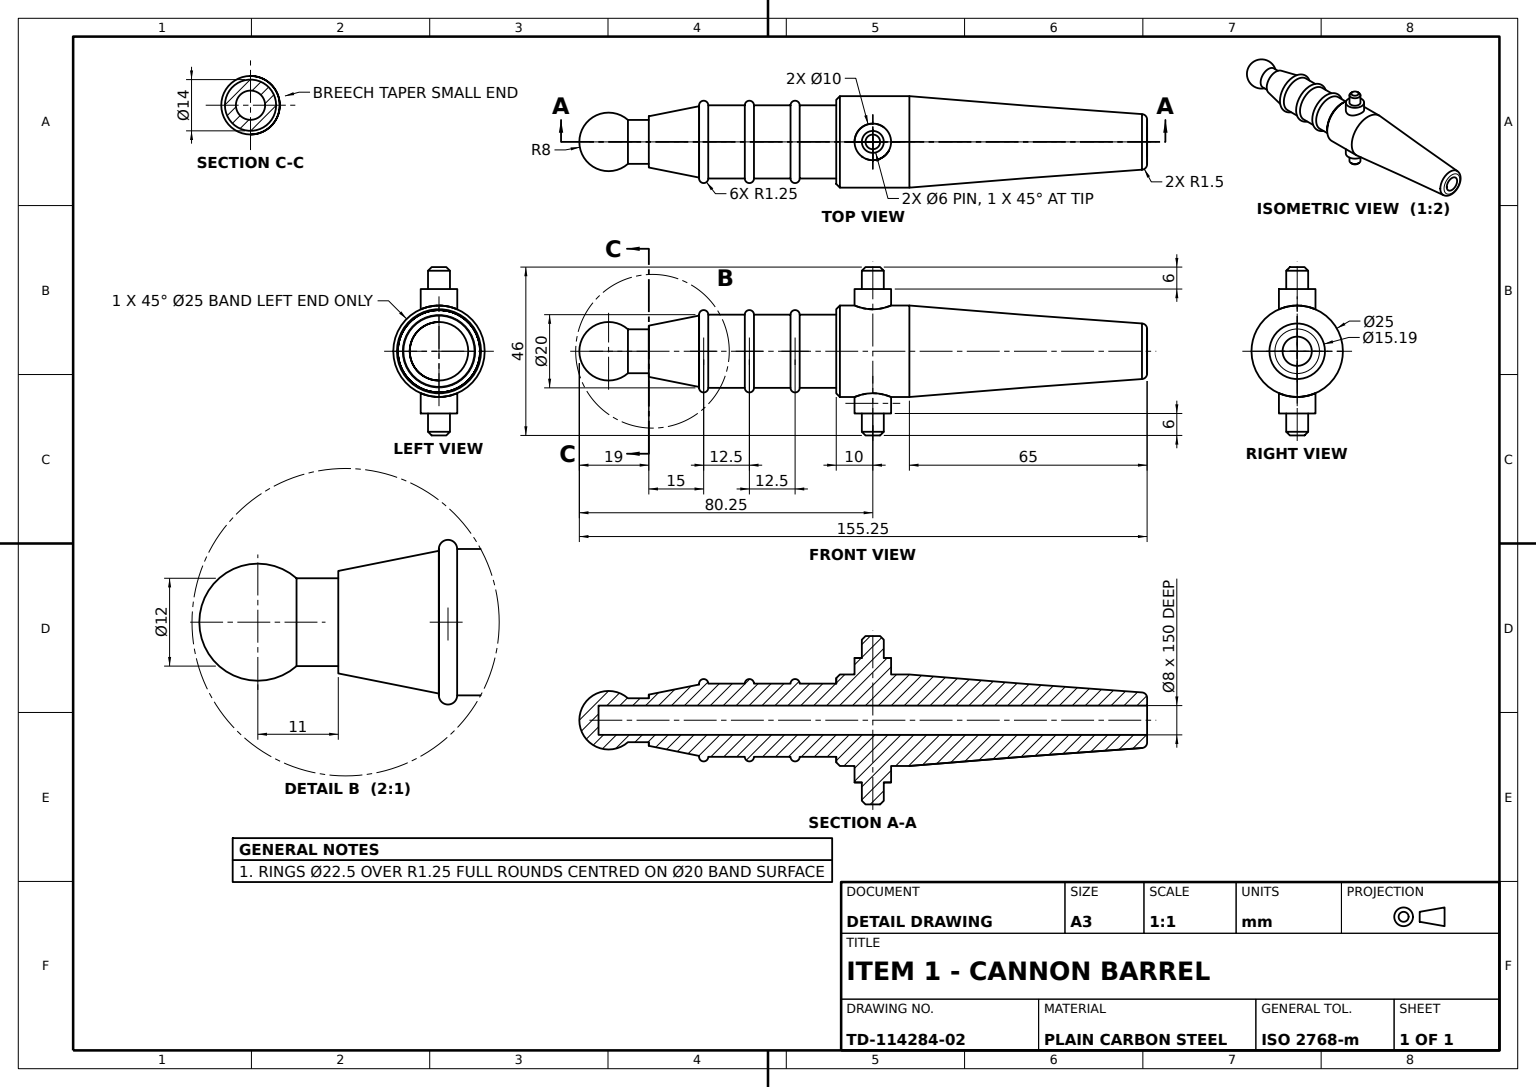
ISO-10303-21;
HEADER;
FILE_DESCRIPTION((''),'2;1');
FILE_NAME('','',(''),(''),'','','');
FILE_SCHEMA(('AUTOMOTIVE_DESIGN'));
ENDSEC;
DATA;
#1=APPLICATION_CONTEXT('');
#2=PRODUCT_CONTEXT('',#1,'mechanical');
#3=PRODUCT('','','',(#2));
#4=PRODUCT_DEFINITION_FORMATION('','',#3);
#5=PRODUCT_DEFINITION_CONTEXT('',#1,'design');
#6=PRODUCT_DEFINITION('','',#4,#5);
#7=PRODUCT_DEFINITION_SHAPE('','',#6);
#8=(LENGTH_UNIT()NAMED_UNIT(*)SI_UNIT(.MILLI.,.METRE.));
#9=(NAMED_UNIT(*)PLANE_ANGLE_UNIT()SI_UNIT($,.RADIAN.));
#10=(NAMED_UNIT(*)SI_UNIT($,.STERADIAN.)SOLID_ANGLE_UNIT());
#11=UNCERTAINTY_MEASURE_WITH_UNIT(LENGTH_MEASURE(1.E-05),#8,'distance_accuracy_value','');
#12=(GEOMETRIC_REPRESENTATION_CONTEXT(3)GLOBAL_UNCERTAINTY_ASSIGNED_CONTEXT((#11))GLOBAL_UNIT_ASSIGNED_CONTEXT((#8,#9,#10))REPRESENTATION_CONTEXT('',''));
#13=CARTESIAN_POINT('',(80.25,-17.,-3.));
#14=VERTEX_POINT('',#13);
#15=CARTESIAN_POINT('',(80.25,-17.,3.));
#16=VERTEX_POINT('',#15);
#17=CARTESIAN_POINT('',(80.25,-17.,0.));
#18=DIRECTION('',(0.,1.,0.));
#19=DIRECTION('',(0.,0.,1.));
#20=AXIS2_PLACEMENT_3D('',#17,#18,#19);
#21=CIRCLE('',#20,3.);
#22=EDGE_CURVE('',#14,#16,#21,.T.);
#23=ORIENTED_EDGE('',*,*,#22,.F.);
#24=CARTESIAN_POINT('',(80.25,-22.,-3.));
#25=VERTEX_POINT('',#24);
#26=CARTESIAN_POINT('',(80.25,-23.,-3.));
#27=VECTOR('',#18,1000.);
#28=LINE('',#26,#27);
#29=EDGE_CURVE('',#25,#14,#28,.T.);
#30=ORIENTED_EDGE('',*,*,#29,.F.);
#31=CARTESIAN_POINT('',(80.25,-22.,3.));
#32=VERTEX_POINT('',#31);
#33=CARTESIAN_POINT('',(80.25,-22.,0.));
#34=DIRECTION('',(0.,0.,-1.));
#35=AXIS2_PLACEMENT_3D('',#33,#18,#34);
#36=CIRCLE('',#35,3.);
#37=EDGE_CURVE('',#25,#32,#36,.T.);
#38=ORIENTED_EDGE('',*,*,#37,.T.);
#39=CARTESIAN_POINT('',(80.25,-23.,3.));
#40=LINE('',#39,#27);
#41=EDGE_CURVE('',#32,#16,#40,.T.);
#42=ORIENTED_EDGE('',*,*,#41,.T.);
#43=EDGE_LOOP('',(#23,#30,#38,#42));
#44=FACE_OUTER_BOUND('',#43,.T.);
#45=CARTESIAN_POINT('',(80.25,-23.,0.));
#46=AXIS2_PLACEMENT_3D('',#45,#18,#34);
#47=CYLINDRICAL_SURFACE('',#46,3.);
#48=ADVANCED_FACE('',(#44),#47,.T.);
#49=CARTESIAN_POINT('',(57.75,0.,-10.));
#50=VERTEX_POINT('',#49);
#51=CARTESIAN_POINT('',(60.25,0.,-10.));
#52=VERTEX_POINT('',#51);
#53=CARTESIAN_POINT('',(59.,0.,-10.));
#54=DIRECTION('',(0.,-1.,0.));
#55=AXIS2_PLACEMENT_3D('',#53,#54,#34);
#56=CIRCLE('',#55,1.25);
#57=EDGE_CURVE('',#50,#52,#56,.T.);
#58=ORIENTED_EDGE('',*,*,#57,.T.);
#59=CARTESIAN_POINT('',(60.25,0.,10.));
#60=VERTEX_POINT('',#59);
#61=CARTESIAN_POINT('',(60.25,0.,0.));
#62=DIRECTION('',(1.,0.,0.));
#63=AXIS2_PLACEMENT_3D('',#61,#62,#34);
#64=CIRCLE('',#63,10.);
#65=EDGE_CURVE('',#60,#52,#64,.T.);
#66=ORIENTED_EDGE('',*,*,#65,.F.);
#67=CARTESIAN_POINT('',(57.75,0.,10.));
#68=VERTEX_POINT('',#67);
#69=CARTESIAN_POINT('',(59.,0.,10.));
#70=AXIS2_PLACEMENT_3D('',#69,#18,#19);
#71=CIRCLE('',#70,1.25);
#72=EDGE_CURVE('',#68,#60,#71,.T.);
#73=ORIENTED_EDGE('',*,*,#72,.F.);
#74=CARTESIAN_POINT('',(57.75,0.,0.));
#75=AXIS2_PLACEMENT_3D('',#74,#62,#34);
#76=CIRCLE('',#75,10.);
#77=EDGE_CURVE('',#68,#50,#76,.T.);
#78=ORIENTED_EDGE('',*,*,#77,.T.);
#79=EDGE_LOOP('',(#58,#66,#73,#78));
#80=FACE_OUTER_BOUND('',#79,.T.);
#81=CARTESIAN_POINT('',(59.,0.,0.));
#82=AXIS2_PLACEMENT_3D('',#81,#62,#34);
#83=TOROIDAL_SURFACE('',#82,10.,1.25);
#84=ADVANCED_FACE('',(#80),#83,.T.);
#85=EDGE_CURVE('',#52,#60,#64,.T.);
#86=ORIENTED_EDGE('',*,*,#85,.T.);
#87=CARTESIAN_POINT('',(70.25,0.,10.));
#88=VERTEX_POINT('',#87);
#89=DIRECTION('',(-1.,0.,0.));
#90=VECTOR('',#89,1000.);
#91=LINE('',#87,#90);
#92=EDGE_CURVE('',#88,#60,#91,.T.);
#93=ORIENTED_EDGE('',*,*,#92,.F.);
#94=CARTESIAN_POINT('',(70.25,0.,-10.));
#95=VERTEX_POINT('',#94);
#96=CARTESIAN_POINT('',(70.25,0.,0.));
#97=AXIS2_PLACEMENT_3D('',#96,#62,#34);
#98=CIRCLE('',#97,10.);
#99=EDGE_CURVE('',#95,#88,#98,.T.);
#100=ORIENTED_EDGE('',*,*,#99,.F.);
#101=LINE('',#94,#90);
#102=EDGE_CURVE('',#95,#52,#101,.T.);
#103=ORIENTED_EDGE('',*,*,#102,.T.);
#104=EDGE_LOOP('',(#86,#93,#100,#103));
#105=FACE_OUTER_BOUND('',#104,.T.);
#106=AXIS2_PLACEMENT_3D('',#96,#89,#19);
#107=CYLINDRICAL_SURFACE('',#106,10.);
#108=ADVANCED_FACE('',(#105),#107,.T.);
#109=CARTESIAN_POINT('',(155.25,0.,6.096209));
#110=VERTEX_POINT('',#109);
#111=CARTESIAN_POINT('',(155.25,0.,-6.096209));
#112=VERTEX_POINT('',#111);
#113=CARTESIAN_POINT('',(155.25,0.,0.));
#114=AXIS2_PLACEMENT_3D('',#113,#62,#34);
#115=CIRCLE('',#114,6.096209);
#116=EDGE_CURVE('',#110,#112,#115,.T.);
#117=ORIENTED_EDGE('',*,*,#116,.F.);
#118=CARTESIAN_POINT('',(153.849844,0.,7.592883));
#119=VERTEX_POINT('',#118);
#120=CARTESIAN_POINT('',(153.75,0.,6.096209));
#121=AXIS2_PLACEMENT_3D('',#120,#18,#19);
#122=CIRCLE('',#121,1.5);
#123=EDGE_CURVE('',#119,#110,#122,.T.);
#124=ORIENTED_EDGE('',*,*,#123,.F.);
#125=CARTESIAN_POINT('',(153.849844,-1.215038,-7.495035));
#126=VERTEX_POINT('',#125);
#127=CARTESIAN_POINT('',(153.849844,0.,0.));
#128=AXIS2_PLACEMENT_3D('',#127,#89,#34);
#129=CIRCLE('',#128,7.592883);
#130=EDGE_CURVE('',#126,#119,#129,.T.);
#131=ORIENTED_EDGE('',*,*,#130,.F.);
#132=CARTESIAN_POINT('',(153.849844,0.,-7.592883));
#133=VERTEX_POINT('',#132);
#134=EDGE_CURVE('',#133,#126,#129,.T.);
#135=ORIENTED_EDGE('',*,*,#134,.F.);
#136=CARTESIAN_POINT('',(153.75,0.,-6.096209));
#137=AXIS2_PLACEMENT_3D('',#136,#54,#34);
#138=CIRCLE('',#137,1.5);
#139=EDGE_CURVE('',#133,#112,#138,.T.);
#140=ORIENTED_EDGE('',*,*,#139,.T.);
#141=EDGE_LOOP('',(#117,#124,#131,#135,#140));
#142=FACE_OUTER_BOUND('',#141,.T.);
#143=CARTESIAN_POINT('',(153.75,0.,0.));
#144=AXIS2_PLACEMENT_3D('',#143,#62,#34);
#145=TOROIDAL_SURFACE('',#144,6.096209,1.5);
#146=ADVANCED_FACE('',(#142),#145,.T.);
#147=CARTESIAN_POINT('',(19.,0.,-7.));
#148=VERTEX_POINT('',#147);
#149=CARTESIAN_POINT('',(19.,0.,7.));
#150=VERTEX_POINT('',#149);
#151=CARTESIAN_POINT('',(19.,0.,0.));
#152=AXIS2_PLACEMENT_3D('',#151,#62,#34);
#153=CIRCLE('',#152,7.);
#154=EDGE_CURVE('',#148,#150,#153,.T.);
#155=ORIENTED_EDGE('',*,*,#154,.T.);
#156=CARTESIAN_POINT('',(32.75,0.,9.75));
#157=VERTEX_POINT('',#156);
#158=DIRECTION('',(0.980580676,0.,0.196116135));
#159=VECTOR('',#158,1000.);
#160=LINE('',#149,#159);
#161=EDGE_CURVE('',#150,#157,#160,.T.);
#162=ORIENTED_EDGE('',*,*,#161,.T.);
#163=CARTESIAN_POINT('',(32.75,0.,-9.75));
#164=VERTEX_POINT('',#163);
#165=CARTESIAN_POINT('',(32.75,0.,0.));
#166=AXIS2_PLACEMENT_3D('',#165,#89,#34);
#167=CIRCLE('',#166,9.75);
#168=EDGE_CURVE('',#157,#164,#167,.T.);
#169=ORIENTED_EDGE('',*,*,#168,.T.);
#170=DIRECTION('',(0.980580676,0.,-0.196116135));
#171=VECTOR('',#170,1000.);
#172=LINE('',#147,#171);
#173=EDGE_CURVE('',#148,#164,#172,.T.);
#174=ORIENTED_EDGE('',*,*,#173,.F.);
#175=EDGE_LOOP('',(#155,#162,#169,#174));
#176=FACE_OUTER_BOUND('',#175,.T.);
#177=CONICAL_SURFACE('',#152,7.,0.19739556);
#178=ADVANCED_FACE('',(#176),#177,.T.);
#179=CARTESIAN_POINT('',(32.75,0.,-10.));
#180=VERTEX_POINT('',#179);
#181=CARTESIAN_POINT('',(32.75,0.,10.));
#182=VERTEX_POINT('',#181);
#183=CIRCLE('',#166,10.);
#184=EDGE_CURVE('',#180,#182,#183,.T.);
#185=ORIENTED_EDGE('',*,*,#184,.T.);
#186=EDGE_CURVE('',#182,#180,#183,.T.);
#187=ORIENTED_EDGE('',*,*,#186,.T.);
#188=EDGE_LOOP('',(#185,#187));
#189=FACE_OUTER_BOUND('',#188,.T.);
#190=EDGE_CURVE('',#164,#157,#167,.T.);
#191=ORIENTED_EDGE('',*,*,#190,.F.);
#192=ORIENTED_EDGE('',*,*,#168,.F.);
#193=EDGE_LOOP('',(#191,#192));
#194=FACE_BOUND('',#193,.T.);
#195=AXIS2_PLACEMENT_3D('',#165,#62,#34);
#196=PLANE('',#195);
#197=ADVANCED_FACE('',(#189,#194),#196,.F.);
#198=CARTESIAN_POINT('',(45.25,0.,10.));
#199=VERTEX_POINT('',#198);
#200=CARTESIAN_POINT('',(47.75,0.,10.));
#201=VERTEX_POINT('',#200);
#202=CARTESIAN_POINT('',(46.5,0.,10.));
#203=AXIS2_PLACEMENT_3D('',#202,#18,#19);
#204=CIRCLE('',#203,1.25);
#205=EDGE_CURVE('',#199,#201,#204,.T.);
#206=ORIENTED_EDGE('',*,*,#205,.F.);
#207=CARTESIAN_POINT('',(45.25,0.,-10.));
#208=VERTEX_POINT('',#207);
#209=CARTESIAN_POINT('',(45.25,0.,0.));
#210=AXIS2_PLACEMENT_3D('',#209,#62,#34);
#211=CIRCLE('',#210,10.);
#212=EDGE_CURVE('',#199,#208,#211,.T.);
#213=ORIENTED_EDGE('',*,*,#212,.T.);
#214=CARTESIAN_POINT('',(47.75,0.,-10.));
#215=VERTEX_POINT('',#214);
#216=CARTESIAN_POINT('',(46.5,0.,-10.));
#217=AXIS2_PLACEMENT_3D('',#216,#54,#34);
#218=CIRCLE('',#217,1.25);
#219=EDGE_CURVE('',#208,#215,#218,.T.);
#220=ORIENTED_EDGE('',*,*,#219,.T.);
#221=CARTESIAN_POINT('',(47.75,0.,0.));
#222=AXIS2_PLACEMENT_3D('',#221,#62,#34);
#223=CIRCLE('',#222,10.);
#224=EDGE_CURVE('',#201,#215,#223,.T.);
#225=ORIENTED_EDGE('',*,*,#224,.F.);
#226=EDGE_LOOP('',(#206,#213,#220,#225));
#227=FACE_OUTER_BOUND('',#226,.T.);
#228=CARTESIAN_POINT('',(46.5,0.,0.));
#229=AXIS2_PLACEMENT_3D('',#228,#62,#34);
#230=TOROIDAL_SURFACE('',#229,10.,1.25);
#231=ADVANCED_FACE('',(#227),#230,.T.);
#232=CARTESIAN_POINT('',(80.25,23.,-2.));
#233=VERTEX_POINT('',#232);
#234=CARTESIAN_POINT('',(80.25,23.,2.));
#235=VERTEX_POINT('',#234);
#236=CARTESIAN_POINT('',(80.25,23.,0.));
#237=AXIS2_PLACEMENT_3D('',#236,#18,#19);
#238=CIRCLE('',#237,2.);
#239=EDGE_CURVE('',#233,#235,#238,.T.);
#240=ORIENTED_EDGE('',*,*,#239,.T.);
#241=EDGE_CURVE('',#235,#233,#238,.T.);
#242=ORIENTED_EDGE('',*,*,#241,.T.);
#243=EDGE_LOOP('',(#240,#242));
#244=FACE_OUTER_BOUND('',#243,.T.);
#245=PLANE('',#237);
#246=ADVANCED_FACE('',(#244),#245,.T.);
#247=CARTESIAN_POINT('',(80.25,17.,5.));
#248=VERTEX_POINT('',#247);
#249=CARTESIAN_POINT('',(80.25,17.,-5.));
#250=VERTEX_POINT('',#249);
#251=CARTESIAN_POINT('',(80.25,17.,0.));
#252=AXIS2_PLACEMENT_3D('',#251,#18,#19);
#253=CIRCLE('',#252,5.);
#254=EDGE_CURVE('',#248,#250,#253,.T.);
#255=ORIENTED_EDGE('',*,*,#254,.T.);
#256=EDGE_CURVE('',#250,#248,#253,.T.);
#257=ORIENTED_EDGE('',*,*,#256,.T.);
#258=EDGE_LOOP('',(#255,#257));
#259=FACE_OUTER_BOUND('',#258,.T.);
#260=CARTESIAN_POINT('',(80.25,17.,-3.));
#261=VERTEX_POINT('',#260);
#262=CARTESIAN_POINT('',(80.25,17.,3.));
#263=VERTEX_POINT('',#262);
#264=CIRCLE('',#252,3.);
#265=EDGE_CURVE('',#261,#263,#264,.T.);
#266=ORIENTED_EDGE('',*,*,#265,.F.);
#267=EDGE_CURVE('',#263,#261,#264,.T.);
#268=ORIENTED_EDGE('',*,*,#267,.F.);
#269=EDGE_LOOP('',(#266,#268));
#270=FACE_BOUND('',#269,.T.);
#271=PLANE('',#252);
#272=ADVANCED_FACE('',(#259,#270),#271,.T.);
#273=CARTESIAN_POINT('',(80.25,-23.,2.));
#274=VERTEX_POINT('',#273);
#275=DIRECTION('',(0.,0.707106781,0.707106781));
#276=VECTOR('',#275,1000.);
#277=LINE('',#31,#276);
#278=EDGE_CURVE('',#274,#32,#277,.T.);
#279=ORIENTED_EDGE('',*,*,#278,.F.);
#280=CARTESIAN_POINT('',(80.25,-23.,-2.));
#281=VERTEX_POINT('',#280);
#282=AXIS2_PLACEMENT_3D('',#45,#54,#34);
#283=CIRCLE('',#282,2.);
#284=EDGE_CURVE('',#281,#274,#283,.T.);
#285=ORIENTED_EDGE('',*,*,#284,.F.);
#286=DIRECTION('',(0.,0.707106781,-0.707106781));
#287=VECTOR('',#286,1000.);
#288=LINE('',#24,#287);
#289=EDGE_CURVE('',#281,#25,#288,.T.);
#290=ORIENTED_EDGE('',*,*,#289,.T.);
#291=EDGE_CURVE('',#32,#25,#36,.T.);
#292=ORIENTED_EDGE('',*,*,#291,.F.);
#293=EDGE_LOOP('',(#279,#285,#290,#292));
#294=FACE_OUTER_BOUND('',#293,.T.);
#295=AXIS2_PLACEMENT_3D('',#33,#18,#19);
#296=CONICAL_SURFACE('',#295,3.,0.785398163);
#297=ADVANCED_FACE('',(#294),#296,.T.);
#298=CARTESIAN_POINT('',(80.25,-17.,-5.));
#299=VERTEX_POINT('',#298);
#300=CARTESIAN_POINT('',(80.25,-11.456439,-5.));
#301=VERTEX_POINT('',#300);
#302=LINE('',#298,#27);
#303=EDGE_CURVE('',#299,#301,#302,.T.);
#304=ORIENTED_EDGE('',*,*,#303,.F.);
#305=CARTESIAN_POINT('',(80.25,-17.,5.));
#306=VERTEX_POINT('',#305);
#307=CIRCLE('',#20,5.);
#308=EDGE_CURVE('',#299,#306,#307,.T.);
#309=ORIENTED_EDGE('',*,*,#308,.T.);
#310=CARTESIAN_POINT('',(80.25,-11.456439,5.));
#311=VERTEX_POINT('',#310);
#312=LINE('',#305,#27);
#313=EDGE_CURVE('',#306,#311,#312,.T.);
#314=ORIENTED_EDGE('',*,*,#313,.T.);
#315=CARTESIAN_POINT('',(80.085653,-11.456439,5.));
#316=CARTESIAN_POINT('',(79.921145,-11.459977,4.991917));
#317=CARTESIAN_POINT('',(79.591799,-11.474152,4.95925));
#318=CARTESIAN_POINT('',(79.426246,-11.484883,4.934441));
#319=CARTESIAN_POINT('',(78.940503,-11.526521,4.836768));
#320=CARTESIAN_POINT('',(78.627856,-11.566876,4.74086));
#321=CARTESIAN_POINT('',(78.023716,-11.666945,4.488961));
#322=CARTESIAN_POINT('',(77.73313,-11.726743,4.332438));
#323=CARTESIAN_POINT('',(77.195837,-11.853682,3.971994));
#324=CARTESIAN_POINT('',(76.944945,-11.921614,3.766013));
#325=CARTESIAN_POINT('',(76.483996,-12.057541,3.305064));
#326=CARTESIAN_POINT('',(76.27914,-12.123902,3.055624));
#327=CARTESIAN_POINT('',(76.008759,-12.216012,2.652925));
#328=CARTESIAN_POINT('',(75.924833,-12.245482,2.5139));
#329=CARTESIAN_POINT('',(75.769754,-12.301112,2.225795));
#330=CARTESIAN_POINT('',(75.698612,-12.327275,2.076452));
#331=CARTESIAN_POINT('',(75.50956,-12.397907,1.623375));
#332=CARTESIAN_POINT('',(75.41384,-12.435227,1.31136));
#333=CARTESIAN_POINT('',(75.283759,-12.486392,0.666754));
#334=CARTESIAN_POINT('',(75.250149,-12.499941,0.331694));
#335=CARTESIAN_POINT('',(75.249852,-12.500059,-0.3272));
#336=CARTESIAN_POINT('',(75.281945,-12.487113,-0.654789));
#337=CARTESIAN_POINT('',(75.412211,-12.43586,-1.306183));
#338=CARTESIAN_POINT('',(75.508963,-12.39814,-1.621438));
#339=CARTESIAN_POINT('',(75.759943,-12.304351,-2.223935));
#340=CARTESIAN_POINT('',(75.916604,-12.247421,-2.515429));
#341=CARTESIAN_POINT('',(76.278847,-12.123987,-3.05543));
#342=CARTESIAN_POINT('',(76.483867,-12.057604,-3.304746));
#343=CARTESIAN_POINT('',(76.942164,-11.922409,-3.76342));
#344=CARTESIAN_POINT('',(77.195641,-11.853742,-3.971801));
#345=CARTESIAN_POINT('',(77.732017,-11.726992,-4.331752));
#346=CARTESIAN_POINT('',(78.017216,-11.668143,-4.485881));
#347=CARTESIAN_POINT('',(78.624871,-11.56725,-4.73998));
#348=CARTESIAN_POINT('',(78.939575,-11.526683,-4.836378));
#349=CARTESIAN_POINT('',(79.583163,-11.471351,-4.966195));
#350=CARTESIAN_POINT('',(79.916115,-11.456439,-5.));
#351=B_SPLINE_CURVE_WITH_KNOTS('',3,(#310,#315,#316,#317,#318,#319,#320,#321,#322,#323,#324,#325,#326,#327,#328,#329,#330,#331,#332,#333,#334,#335,#336,#337,#338,#339,#340,#341,#342,#343,#344,#345,#346,#347,#348,#349,#350,#300),.UNSPECIFIED.,.F.,.F.,(4,2,2,2,2,2,2,2,2,2,2,2,2,2,2,2,2,2,4),(0.015798618,0.016291875,0.016785132,0.017771645,0.018758159,0.019744672,0.020731186,0.021224442,0.021717699,0.022704212,0.023690726,0.024677239,0.025663753,0.026650266,0.02763678,0.028623293,0.029609806,0.03059632,0.031582833),.UNSPECIFIED.);
#352=EDGE_CURVE('',#311,#301,#351,.T.);
#353=ORIENTED_EDGE('',*,*,#352,.T.);
#354=EDGE_LOOP('',(#304,#309,#314,#353));
#355=FACE_OUTER_BOUND('',#354,.T.);
#356=AXIS2_PLACEMENT_3D('',#17,#18,#34);
#357=CYLINDRICAL_SURFACE('',#356,5.);
#358=ADVANCED_FACE('',(#355),#357,.T.);
#359=ORIENTED_EDGE('',*,*,#224,.T.);
#360=LINE('',#49,#90);
#361=EDGE_CURVE('',#50,#215,#360,.T.);
#362=ORIENTED_EDGE('',*,*,#361,.F.);
#363=ORIENTED_EDGE('',*,*,#77,.F.);
#364=LINE('',#67,#90);
#365=EDGE_CURVE('',#68,#201,#364,.T.);
#366=ORIENTED_EDGE('',*,*,#365,.T.);
#367=EDGE_LOOP('',(#359,#362,#363,#366));
#368=FACE_OUTER_BOUND('',#367,.T.);
#369=AXIS2_PLACEMENT_3D('',#74,#89,#19);
#370=CYLINDRICAL_SURFACE('',#369,10.);
#371=ADVANCED_FACE('',(#368),#370,.T.);
#372=CARTESIAN_POINT('',(5.25,0.,4.));
#373=VERTEX_POINT('',#372);
#374=CARTESIAN_POINT('',(155.25,0.,4.));
#375=VERTEX_POINT('',#374);
#376=VECTOR('',#62,1000.);
#377=LINE('',#372,#376);
#378=EDGE_CURVE('',#373,#375,#377,.T.);
#379=ORIENTED_EDGE('',*,*,#378,.F.);
#380=CARTESIAN_POINT('',(5.25,0.,-4.));
#381=VERTEX_POINT('',#380);
#382=CARTESIAN_POINT('',(5.25,0.,0.));
#383=AXIS2_PLACEMENT_3D('',#382,#62,#34);
#384=CIRCLE('',#383,4.);
#385=EDGE_CURVE('',#381,#373,#384,.T.);
#386=ORIENTED_EDGE('',*,*,#385,.F.);
#387=CARTESIAN_POINT('',(155.25,0.,-4.));
#388=VERTEX_POINT('',#387);
#389=LINE('',#380,#376);
#390=EDGE_CURVE('',#381,#388,#389,.T.);
#391=ORIENTED_EDGE('',*,*,#390,.T.);
#392=CIRCLE('',#114,4.);
#393=EDGE_CURVE('',#388,#375,#392,.T.);
#394=ORIENTED_EDGE('',*,*,#393,.T.);
#395=EDGE_LOOP('',(#379,#386,#391,#394));
#396=FACE_OUTER_BOUND('',#395,.T.);
#397=CYLINDRICAL_SURFACE('',#383,4.);
#398=ADVANCED_FACE('',(#396),#397,.F.);
#399=CARTESIAN_POINT('',(19.,0.,-6.));
#400=VERTEX_POINT('',#399);
#401=CARTESIAN_POINT('',(19.,0.,6.));
#402=VERTEX_POINT('',#401);
#403=CIRCLE('',#152,6.);
#404=EDGE_CURVE('',#400,#402,#403,.T.);
#405=ORIENTED_EDGE('',*,*,#404,.T.);
#406=EDGE_CURVE('',#402,#400,#403,.T.);
#407=ORIENTED_EDGE('',*,*,#406,.T.);
#408=EDGE_LOOP('',(#405,#407));
#409=FACE_BOUND('',#408,.T.);
#410=EDGE_CURVE('',#150,#148,#153,.T.);
#411=ORIENTED_EDGE('',*,*,#410,.F.);
#412=ORIENTED_EDGE('',*,*,#154,.F.);
#413=EDGE_LOOP('',(#411,#412));
#414=FACE_OUTER_BOUND('',#413,.T.);
#415=PLANE('',#152);
#416=ADVANCED_FACE('',(#409,#414),#415,.F.);
#417=CARTESIAN_POINT('',(13.291503,0.,6.));
#418=VERTEX_POINT('',#417);
#419=LINE('',#401,#90);
#420=EDGE_CURVE('',#402,#418,#419,.T.);
#421=ORIENTED_EDGE('',*,*,#420,.F.);
#422=ORIENTED_EDGE('',*,*,#404,.F.);
#423=CARTESIAN_POINT('',(13.291503,0.,-6.));
#424=VERTEX_POINT('',#423);
#425=LINE('',#399,#90);
#426=EDGE_CURVE('',#400,#424,#425,.T.);
#427=ORIENTED_EDGE('',*,*,#426,.T.);
#428=CARTESIAN_POINT('',(13.291503,0.,0.));
#429=AXIS2_PLACEMENT_3D('',#428,#62,#19);
#430=CIRCLE('',#429,6.);
#431=EDGE_CURVE('',#424,#418,#430,.T.);
#432=ORIENTED_EDGE('',*,*,#431,.T.);
#433=EDGE_LOOP('',(#421,#422,#427,#432));
#434=FACE_OUTER_BOUND('',#433,.T.);
#435=AXIS2_PLACEMENT_3D('',#151,#89,#19);
#436=CYLINDRICAL_SURFACE('',#435,6.);
#437=ADVANCED_FACE('',(#434),#436,.T.);
#438=ORIENTED_EDGE('',*,*,#352,.F.);
#439=CARTESIAN_POINT('',(80.584189,-11.456439,-5.));
#440=CARTESIAN_POINT('',(80.912005,-11.471069,-4.96684));
#441=CARTESIAN_POINT('',(81.555686,-11.526144,-4.837658));
#442=CARTESIAN_POINT('',(81.874909,-11.567272,-4.739896));
#443=CARTESIAN_POINT('',(82.478447,-11.667365,-4.487869));
#444=CARTESIAN_POINT('',(82.764133,-11.726118,-4.334177));
#445=CARTESIAN_POINT('',(83.304847,-11.853821,-3.971632));
#446=CARTESIAN_POINT('',(83.557685,-11.922386,-3.763409));
#447=CARTESIAN_POINT('',(84.013789,-12.056891,-3.307252));
#448=CARTESIAN_POINT('',(84.220371,-12.123715,-3.056682));
#449=CARTESIAN_POINT('',(84.585008,-12.247976,-2.512938));
#450=CARTESIAN_POINT('',(84.738544,-12.3038,-2.226869));
#451=CARTESIAN_POINT('',(84.926683,-12.374085,-1.776268));
#452=CARTESIAN_POINT('',(84.982313,-12.395273,-1.62246));
#453=CARTESIAN_POINT('',(85.078892,-12.432466,-1.307275));
#454=CARTESIAN_POINT('',(85.119847,-12.448475,-1.145353));
#455=CARTESIAN_POINT('',(85.217254,-12.486795,-0.659831));
#456=CARTESIAN_POINT('',(85.249829,-12.499932,-0.332863));
#457=CARTESIAN_POINT('',(85.25017,-12.500068,0.327703));
#458=CARTESIAN_POINT('',(85.21678,-12.486607,0.662722));
#459=CARTESIAN_POINT('',(85.087224,-12.435642,1.307428));
#460=CARTESIAN_POINT('',(84.991299,-12.398224,1.621509));
#461=CARTESIAN_POINT('',(84.736648,-12.303091,2.231412));
#462=CARTESIAN_POINT('',(84.581972,-12.246922,2.51777));
#463=CARTESIAN_POINT('',(84.220477,-12.12377,3.056217));
#464=CARTESIAN_POINT('',(84.011131,-12.056043,3.310386));
#465=CARTESIAN_POINT('',(83.552942,-11.921053,3.76767));
#466=CARTESIAN_POINT('',(83.303839,-11.85357,3.972364));
#467=CARTESIAN_POINT('',(82.763955,-11.726089,4.33424));
#468=CARTESIAN_POINT('',(82.472914,-11.666349,4.490479));
#469=CARTESIAN_POINT('',(81.872549,-11.56698,4.740578));
#470=CARTESIAN_POINT('',(81.560267,-11.526561,4.836676));
#471=CARTESIAN_POINT('',(80.909238,-11.470807,4.967458));
#472=CARTESIAN_POINT('',(80.578994,-11.456439,5.));
#473=B_SPLINE_CURVE_WITH_KNOTS('',3,(#300,#439,#440,#441,#442,#443,#444,#445,#446,#447,#448,#449,#450,#451,#452,#453,#454,#455,#456,#457,#458,#459,#460,#461,#462,#463,#464,#465,#466,#467,#468,#469,#470,#471,#472,#310),.UNSPECIFIED.,.F.,.F.,(4,2,2,2,2,2,2,2,2,2,2,2,2,2,2,2,2,4),(0.,0.000987414,0.001974827,0.002962241,0.003949655,0.004937068,0.005924482,0.006418189,0.006911896,0.007899309,0.008886723,0.009874137,0.01086155,0.011848964,0.012836377,0.013823791,0.014811205,0.015798618),.UNSPECIFIED.);
#474=EDGE_CURVE('',#301,#311,#473,.T.);
#475=ORIENTED_EDGE('',*,*,#474,.F.);
#476=EDGE_LOOP('',(#438,#475));
#477=FACE_BOUND('',#476,.T.);
#478=CARTESIAN_POINT('',(71.25,0.,12.5));
#479=VERTEX_POINT('',#478);
#480=CARTESIAN_POINT('',(71.25,0.,-12.5));
#481=VERTEX_POINT('',#480);
#482=CARTESIAN_POINT('',(71.25,0.,0.));
#483=AXIS2_PLACEMENT_3D('',#482,#62,#34);
#484=CIRCLE('',#483,12.5);
#485=EDGE_CURVE('',#479,#481,#484,.T.);
#486=ORIENTED_EDGE('',*,*,#485,.T.);
#487=CARTESIAN_POINT('',(90.25,0.,-12.5));
#488=VERTEX_POINT('',#487);
#489=LINE('',#487,#90);
#490=EDGE_CURVE('',#488,#481,#489,.T.);
#491=ORIENTED_EDGE('',*,*,#490,.F.);
#492=CARTESIAN_POINT('',(90.25,-5.863,-11.039711));
#493=VERTEX_POINT('',#492);
#494=CARTESIAN_POINT('',(90.25,0.,0.));
#495=AXIS2_PLACEMENT_3D('',#494,#62,#19);
#496=CIRCLE('',#495,12.5);
#497=EDGE_CURVE('',#493,#488,#496,.T.);
#498=ORIENTED_EDGE('',*,*,#497,.F.);
#499=CARTESIAN_POINT('',(90.25,0.,12.5));
#500=VERTEX_POINT('',#499);
#501=EDGE_CURVE('',#500,#493,#496,.T.);
#502=ORIENTED_EDGE('',*,*,#501,.F.);
#503=LINE('',#499,#90);
#504=EDGE_CURVE('',#500,#479,#503,.T.);
#505=ORIENTED_EDGE('',*,*,#504,.T.);
#506=EDGE_LOOP('',(#486,#491,#498,#502,#505));
#507=FACE_OUTER_BOUND('',#506,.T.);
#508=AXIS2_PLACEMENT_3D('',#494,#89,#19);
#509=CYLINDRICAL_SURFACE('',#508,12.5);
#510=ADVANCED_FACE('',(#477,#507),#509,.T.);
#511=EDGE_CURVE('',#274,#281,#283,.T.);
#512=ORIENTED_EDGE('',*,*,#511,.T.);
#513=ORIENTED_EDGE('',*,*,#284,.T.);
#514=EDGE_LOOP('',(#512,#513));
#515=FACE_OUTER_BOUND('',#514,.T.);
#516=AXIS2_PLACEMENT_3D('',#45,#54,#19);
#517=PLANE('',#516);
#518=ADVANCED_FACE('',(#515),#517,.T.);
#519=EDGE_CURVE('',#306,#299,#307,.T.);
#520=ORIENTED_EDGE('',*,*,#519,.F.);
#521=ORIENTED_EDGE('',*,*,#308,.F.);
#522=EDGE_LOOP('',(#520,#521));
#523=FACE_OUTER_BOUND('',#522,.T.);
#524=EDGE_CURVE('',#16,#14,#21,.T.);
#525=ORIENTED_EDGE('',*,*,#524,.T.);
#526=ORIENTED_EDGE('',*,*,#22,.T.);
#527=EDGE_LOOP('',(#525,#526));
#528=FACE_BOUND('',#527,.T.);
#529=AXIS2_PLACEMENT_3D('',#17,#54,#19);
#530=PLANE('',#529);
#531=ADVANCED_FACE('',(#523,#528),#530,.T.);
#532=ORIENTED_EDGE('',*,*,#474,.T.);
#533=ORIENTED_EDGE('',*,*,#313,.F.);
#534=ORIENTED_EDGE('',*,*,#519,.T.);
#535=ORIENTED_EDGE('',*,*,#303,.T.);
#536=EDGE_LOOP('',(#532,#533,#534,#535));
#537=FACE_OUTER_BOUND('',#536,.T.);
#538=ADVANCED_FACE('',(#537),#357,.T.);
#539=ORIENTED_EDGE('',*,*,#219,.F.);
#540=EDGE_CURVE('',#208,#199,#211,.T.);
#541=ORIENTED_EDGE('',*,*,#540,.T.);
#542=ORIENTED_EDGE('',*,*,#205,.T.);
#543=EDGE_CURVE('',#215,#201,#223,.T.);
#544=ORIENTED_EDGE('',*,*,#543,.F.);
#545=EDGE_LOOP('',(#539,#541,#542,#544));
#546=FACE_OUTER_BOUND('',#545,.T.);
#547=ADVANCED_FACE('',(#546),#230,.T.);
#548=ORIENTED_EDGE('',*,*,#361,.T.);
#549=ORIENTED_EDGE('',*,*,#543,.T.);
#550=ORIENTED_EDGE('',*,*,#365,.F.);
#551=EDGE_CURVE('',#50,#68,#76,.T.);
#552=ORIENTED_EDGE('',*,*,#551,.F.);
#553=EDGE_LOOP('',(#548,#549,#550,#552));
#554=FACE_OUTER_BOUND('',#553,.T.);
#555=ADVANCED_FACE('',(#554),#370,.T.);
#556=CARTESIAN_POINT('',(0.,0.,0.));
#557=VERTEX_POINT('',#556);
#558=CARTESIAN_POINT('',(8.,0.,0.));
#559=AXIS2_PLACEMENT_3D('',#558,#54,#34);
#560=CIRCLE('',#559,8.);
#561=EDGE_CURVE('',#418,#557,#560,.T.);
#562=ORIENTED_EDGE('',*,*,#561,.T.);
#563=AXIS2_PLACEMENT_3D('',#558,#18,#19);
#564=CIRCLE('',#563,8.);
#565=EDGE_CURVE('',#424,#557,#564,.T.);
#566=ORIENTED_EDGE('',*,*,#565,.F.);
#567=EDGE_CURVE('',#418,#424,#430,.T.);
#568=ORIENTED_EDGE('',*,*,#567,.F.);
#569=EDGE_LOOP('',(#562,#566,#568));
#570=FACE_OUTER_BOUND('',#569,.T.);
#571=SPHERICAL_SURFACE('',#559,8.);
#572=ADVANCED_FACE('',(#570),#571,.T.);
#573=CARTESIAN_POINT('',(35.25,0.,-10.));
#574=VERTEX_POINT('',#573);
#575=CARTESIAN_POINT('',(34.,0.,-10.));
#576=AXIS2_PLACEMENT_3D('',#575,#54,#34);
#577=CIRCLE('',#576,1.25);
#578=EDGE_CURVE('',#180,#574,#577,.T.);
#579=ORIENTED_EDGE('',*,*,#578,.T.);
#580=CARTESIAN_POINT('',(35.25,0.,10.));
#581=VERTEX_POINT('',#580);
#582=CARTESIAN_POINT('',(35.25,0.,0.));
#583=AXIS2_PLACEMENT_3D('',#582,#62,#34);
#584=CIRCLE('',#583,10.);
#585=EDGE_CURVE('',#581,#574,#584,.T.);
#586=ORIENTED_EDGE('',*,*,#585,.F.);
#587=CARTESIAN_POINT('',(34.,0.,10.));
#588=AXIS2_PLACEMENT_3D('',#587,#18,#19);
#589=CIRCLE('',#588,1.25);
#590=EDGE_CURVE('',#182,#581,#589,.T.);
#591=ORIENTED_EDGE('',*,*,#590,.F.);
#592=ORIENTED_EDGE('',*,*,#184,.F.);
#593=EDGE_LOOP('',(#579,#586,#591,#592));
#594=FACE_OUTER_BOUND('',#593,.T.);
#595=CARTESIAN_POINT('',(34.,0.,0.));
#596=AXIS2_PLACEMENT_3D('',#595,#62,#34);
#597=TOROIDAL_SURFACE('',#596,10.,1.25);
#598=ADVANCED_FACE('',(#594),#597,.T.);
#599=CARTESIAN_POINT('',(80.25,11.456439,5.));
#600=VERTEX_POINT('',#599);
#601=CARTESIAN_POINT('',(80.25,11.456439,-5.));
#602=VERTEX_POINT('',#601);
#603=CARTESIAN_POINT('',(80.414347,11.456439,5.));
#604=CARTESIAN_POINT('',(80.578855,11.459977,4.991917));
#605=CARTESIAN_POINT('',(80.908201,11.474152,4.95925));
#606=CARTESIAN_POINT('',(81.073754,11.484883,4.934441));
#607=CARTESIAN_POINT('',(81.559497,11.526521,4.836768));
#608=CARTESIAN_POINT('',(81.872144,11.566876,4.74086));
#609=CARTESIAN_POINT('',(82.476284,11.666945,4.488961));
#610=CARTESIAN_POINT('',(82.76687,11.726743,4.332438));
#611=CARTESIAN_POINT('',(83.304163,11.853682,3.971994));
#612=CARTESIAN_POINT('',(83.555055,11.921614,3.766013));
#613=CARTESIAN_POINT('',(84.016004,12.057541,3.305064));
#614=CARTESIAN_POINT('',(84.22086,12.123902,3.055624));
#615=CARTESIAN_POINT('',(84.491241,12.216012,2.652925));
#616=CARTESIAN_POINT('',(84.575167,12.245482,2.5139));
#617=CARTESIAN_POINT('',(84.730246,12.301112,2.225795));
#618=CARTESIAN_POINT('',(84.801388,12.327275,2.076452));
#619=CARTESIAN_POINT('',(84.99044,12.397907,1.623375));
#620=CARTESIAN_POINT('',(85.08616,12.435227,1.31136));
#621=CARTESIAN_POINT('',(85.216241,12.486392,0.666754));
#622=CARTESIAN_POINT('',(85.249851,12.499941,0.331694));
#623=CARTESIAN_POINT('',(85.250148,12.500059,-0.3272));
#624=CARTESIAN_POINT('',(85.218055,12.487113,-0.654789));
#625=CARTESIAN_POINT('',(85.087789,12.43586,-1.306183));
#626=CARTESIAN_POINT('',(84.991037,12.39814,-1.621438));
#627=CARTESIAN_POINT('',(84.740057,12.304351,-2.223935));
#628=CARTESIAN_POINT('',(84.583396,12.247421,-2.515429));
#629=CARTESIAN_POINT('',(84.221153,12.123987,-3.05543));
#630=CARTESIAN_POINT('',(84.016133,12.057604,-3.304746));
#631=CARTESIAN_POINT('',(83.557836,11.922409,-3.76342));
#632=CARTESIAN_POINT('',(83.304359,11.853742,-3.971801));
#633=CARTESIAN_POINT('',(82.767983,11.726992,-4.331752));
#634=CARTESIAN_POINT('',(82.482784,11.668143,-4.485881));
#635=CARTESIAN_POINT('',(81.875129,11.56725,-4.73998));
#636=CARTESIAN_POINT('',(81.560425,11.526683,-4.836378));
#637=CARTESIAN_POINT('',(80.916837,11.471351,-4.966195));
#638=CARTESIAN_POINT('',(80.583885,11.456439,-5.));
#639=B_SPLINE_CURVE_WITH_KNOTS('',3,(#599,#603,#604,#605,#606,#607,#608,#609,#610,#611,#612,#613,#614,#615,#616,#617,#618,#619,#620,#621,#622,#623,#624,#625,#626,#627,#628,#629,#630,#631,#632,#633,#634,#635,#636,#637,#638,#601),.UNSPECIFIED.,.F.,.F.,(4,2,2,2,2,2,2,2,2,2,2,2,2,2,2,2,2,2,4),(0.015798618,0.016291875,0.016785132,0.017771645,0.018758159,0.019744672,0.020731186,0.021224442,0.021717699,0.022704212,0.023690726,0.024677239,0.025663753,0.026650266,0.02763678,0.028623293,0.029609806,0.03059632,0.031582833),.UNSPECIFIED.);
#640=EDGE_CURVE('',#600,#602,#639,.T.);
#641=ORIENTED_EDGE('',*,*,#640,.F.);
#642=CARTESIAN_POINT('',(79.915811,11.456439,-5.));
#643=CARTESIAN_POINT('',(79.587995,11.471069,-4.96684));
#644=CARTESIAN_POINT('',(78.944314,11.526144,-4.837658));
#645=CARTESIAN_POINT('',(78.625091,11.567272,-4.739896));
#646=CARTESIAN_POINT('',(78.021553,11.667365,-4.487869));
#647=CARTESIAN_POINT('',(77.735867,11.726118,-4.334177));
#648=CARTESIAN_POINT('',(77.195153,11.853821,-3.971632));
#649=CARTESIAN_POINT('',(76.942315,11.922386,-3.763409));
#650=CARTESIAN_POINT('',(76.486211,12.056891,-3.307252));
#651=CARTESIAN_POINT('',(76.279629,12.123715,-3.056682));
#652=CARTESIAN_POINT('',(75.914992,12.247976,-2.512938));
#653=CARTESIAN_POINT('',(75.761456,12.3038,-2.226869));
#654=CARTESIAN_POINT('',(75.573317,12.374085,-1.776268));
#655=CARTESIAN_POINT('',(75.517687,12.395273,-1.62246));
#656=CARTESIAN_POINT('',(75.421108,12.432466,-1.307275));
#657=CARTESIAN_POINT('',(75.380153,12.448475,-1.145353));
#658=CARTESIAN_POINT('',(75.282746,12.486795,-0.659831));
#659=CARTESIAN_POINT('',(75.250171,12.499932,-0.332863));
#660=CARTESIAN_POINT('',(75.24983,12.500068,0.327703));
#661=CARTESIAN_POINT('',(75.28322,12.486607,0.662722));
#662=CARTESIAN_POINT('',(75.412776,12.435642,1.307428));
#663=CARTESIAN_POINT('',(75.508701,12.398224,1.621509));
#664=CARTESIAN_POINT('',(75.763352,12.303091,2.231412));
#665=CARTESIAN_POINT('',(75.918028,12.246922,2.51777));
#666=CARTESIAN_POINT('',(76.279523,12.12377,3.056217));
#667=CARTESIAN_POINT('',(76.488869,12.056043,3.310386));
#668=CARTESIAN_POINT('',(76.947058,11.921053,3.76767));
#669=CARTESIAN_POINT('',(77.196161,11.85357,3.972364));
#670=CARTESIAN_POINT('',(77.736045,11.726089,4.33424));
#671=CARTESIAN_POINT('',(78.027086,11.666349,4.490479));
#672=CARTESIAN_POINT('',(78.627451,11.56698,4.740578));
#673=CARTESIAN_POINT('',(78.939733,11.526561,4.836676));
#674=CARTESIAN_POINT('',(79.590762,11.470807,4.967458));
#675=CARTESIAN_POINT('',(79.921006,11.456439,5.));
#676=B_SPLINE_CURVE_WITH_KNOTS('',3,(#601,#642,#643,#644,#645,#646,#647,#648,#649,#650,#651,#652,#653,#654,#655,#656,#657,#658,#659,#660,#661,#662,#663,#664,#665,#666,#667,#668,#669,#670,#671,#672,#673,#674,#675,#599),.UNSPECIFIED.,.F.,.F.,(4,2,2,2,2,2,2,2,2,2,2,2,2,2,2,2,2,4),(0.,0.000987414,0.001974827,0.002962241,0.003949655,0.004937068,0.005924482,0.006418189,0.006911896,0.007899309,0.008886723,0.009874137,0.01086155,0.011848964,0.012836377,0.013823791,0.014811205,0.015798618),.UNSPECIFIED.);
#677=EDGE_CURVE('',#602,#600,#676,.T.);
#678=ORIENTED_EDGE('',*,*,#677,.F.);
#679=EDGE_LOOP('',(#641,#678));
#680=FACE_BOUND('',#679,.T.);
#681=CARTESIAN_POINT('',(90.25,5.863,11.039711));
#682=VERTEX_POINT('',#681);
#683=EDGE_CURVE('',#682,#500,#496,.T.);
#684=ORIENTED_EDGE('',*,*,#683,.F.);
#685=EDGE_CURVE('',#488,#682,#496,.T.);
#686=ORIENTED_EDGE('',*,*,#685,.F.);
#687=ORIENTED_EDGE('',*,*,#490,.T.);
#688=EDGE_CURVE('',#481,#479,#484,.T.);
#689=ORIENTED_EDGE('',*,*,#688,.T.);
#690=ORIENTED_EDGE('',*,*,#504,.F.);
#691=EDGE_LOOP('',(#684,#686,#687,#689,#690));
#692=FACE_OUTER_BOUND('',#691,.T.);
#693=ADVANCED_FACE('',(#680,#692),#509,.T.);
#694=ORIENTED_EDGE('',*,*,#190,.T.);
#695=ORIENTED_EDGE('',*,*,#161,.F.);
#696=ORIENTED_EDGE('',*,*,#410,.T.);
#697=ORIENTED_EDGE('',*,*,#173,.T.);
#698=EDGE_LOOP('',(#694,#695,#696,#697));
#699=FACE_OUTER_BOUND('',#698,.T.);
#700=ADVANCED_FACE('',(#699),#177,.T.);
#701=ORIENTED_EDGE('',*,*,#212,.F.);
#702=LINE('',#198,#90);
#703=EDGE_CURVE('',#199,#581,#702,.T.);
#704=ORIENTED_EDGE('',*,*,#703,.T.);
#705=ORIENTED_EDGE('',*,*,#585,.T.);
#706=LINE('',#207,#90);
#707=EDGE_CURVE('',#208,#574,#706,.T.);
#708=ORIENTED_EDGE('',*,*,#707,.F.);
#709=EDGE_LOOP('',(#701,#704,#705,#708));
#710=FACE_OUTER_BOUND('',#709,.T.);
#711=AXIS2_PLACEMENT_3D('',#209,#89,#19);
#712=CYLINDRICAL_SURFACE('',#711,10.);
#713=ADVANCED_FACE('',(#710),#712,.T.);
#714=EDGE_CURVE('',#373,#381,#384,.T.);
#715=ORIENTED_EDGE('',*,*,#714,.F.);
#716=ORIENTED_EDGE('',*,*,#378,.T.);
#717=EDGE_CURVE('',#375,#388,#392,.T.);
#718=ORIENTED_EDGE('',*,*,#717,.T.);
#719=ORIENTED_EDGE('',*,*,#390,.F.);
#720=EDGE_LOOP('',(#715,#716,#718,#719));
#721=FACE_OUTER_BOUND('',#720,.T.);
#722=ADVANCED_FACE('',(#721),#397,.F.);
#723=ORIENTED_EDGE('',*,*,#99,.T.);
#724=EDGE_CURVE('',#88,#95,#98,.T.);
#725=ORIENTED_EDGE('',*,*,#724,.T.);
#726=EDGE_LOOP('',(#723,#725));
#727=FACE_BOUND('',#726,.T.);
#728=CARTESIAN_POINT('',(70.25,0.,-11.5));
#729=VERTEX_POINT('',#728);
#730=CARTESIAN_POINT('',(70.25,0.,11.5));
#731=VERTEX_POINT('',#730);
#732=AXIS2_PLACEMENT_3D('',#96,#89,#34);
#733=CIRCLE('',#732,11.5);
#734=EDGE_CURVE('',#729,#731,#733,.T.);
#735=ORIENTED_EDGE('',*,*,#734,.T.);
#736=EDGE_CURVE('',#731,#729,#733,.T.);
#737=ORIENTED_EDGE('',*,*,#736,.T.);
#738=EDGE_LOOP('',(#735,#737));
#739=FACE_OUTER_BOUND('',#738,.T.);
#740=PLANE('',#97);
#741=ADVANCED_FACE('',(#727,#739),#740,.F.);
#742=CARTESIAN_POINT('',(80.25,22.,3.));
#743=VERTEX_POINT('',#742);
#744=DIRECTION('',(0.,-0.707106781,0.707106781));
#745=VECTOR('',#744,1000.);
#746=LINE('',#234,#745);
#747=EDGE_CURVE('',#235,#743,#746,.T.);
#748=ORIENTED_EDGE('',*,*,#747,.T.);
#749=CARTESIAN_POINT('',(80.25,22.,-3.));
#750=VERTEX_POINT('',#749);
#751=CARTESIAN_POINT('',(80.25,22.,0.));
#752=AXIS2_PLACEMENT_3D('',#751,#54,#19);
#753=CIRCLE('',#752,3.);
#754=EDGE_CURVE('',#750,#743,#753,.T.);
#755=ORIENTED_EDGE('',*,*,#754,.F.);
#756=DIRECTION('',(0.,-0.707106781,-0.707106781));
#757=VECTOR('',#756,1000.);
#758=LINE('',#232,#757);
#759=EDGE_CURVE('',#233,#750,#758,.T.);
#760=ORIENTED_EDGE('',*,*,#759,.F.);
#761=ORIENTED_EDGE('',*,*,#241,.F.);
#762=EDGE_LOOP('',(#748,#755,#760,#761));
#763=FACE_OUTER_BOUND('',#762,.T.);
#764=AXIS2_PLACEMENT_3D('',#236,#54,#34);
#765=CONICAL_SURFACE('',#764,2.,0.785398163);
#766=ADVANCED_FACE('',(#763),#765,.T.);
#767=ORIENTED_EDGE('',*,*,#567,.T.);
#768=ORIENTED_EDGE('',*,*,#426,.F.);
#769=ORIENTED_EDGE('',*,*,#406,.F.);
#770=ORIENTED_EDGE('',*,*,#420,.T.);
#771=EDGE_LOOP('',(#767,#768,#769,#770));
#772=FACE_OUTER_BOUND('',#771,.T.);
#773=ADVANCED_FACE('',(#772),#436,.T.);
#774=ORIENTED_EDGE('',*,*,#393,.F.);
#775=ORIENTED_EDGE('',*,*,#717,.F.);
#776=EDGE_LOOP('',(#774,#775));
#777=FACE_BOUND('',#776,.T.);
#778=EDGE_CURVE('',#112,#110,#115,.T.);
#779=ORIENTED_EDGE('',*,*,#778,.T.);
#780=ORIENTED_EDGE('',*,*,#116,.T.);
#781=EDGE_LOOP('',(#779,#780));
#782=FACE_OUTER_BOUND('',#781,.T.);
#783=PLANE('',#114);
#784=ADVANCED_FACE('',(#777,#782),#783,.T.);
#785=ORIENTED_EDGE('',*,*,#501,.T.);
#786=B_SPLINE_CURVE_WITH_KNOTS('',1,(#492,#125),.UNSPECIFIED.,.F.,.F.,(2,2),(0.,0.978459137),.UNSPECIFIED.);
#787=EDGE_CURVE('',#493,#126,#786,.T.);
#788=ORIENTED_EDGE('',*,*,#787,.T.);
#789=ORIENTED_EDGE('',*,*,#130,.T.);
#790=CARTESIAN_POINT('',(153.849844,1.215038,7.495035));
#791=VERTEX_POINT('',#790);
#792=EDGE_CURVE('',#119,#791,#129,.T.);
#793=ORIENTED_EDGE('',*,*,#792,.T.);
#794=B_SPLINE_CURVE_WITH_KNOTS('',1,(#681,#790),.UNSPECIFIED.,.F.,.F.,(2,2),(0.,0.978459137),.UNSPECIFIED.);
#795=EDGE_CURVE('',#682,#791,#794,.T.);
#796=ORIENTED_EDGE('',*,*,#795,.F.);
#797=ORIENTED_EDGE('',*,*,#683,.T.);
#798=EDGE_LOOP('',(#785,#788,#789,#793,#796,#797));
#799=FACE_OUTER_BOUND('',#798,.T.);
#800=CARTESIAN_POINT('',(155.25,1.112713,7.416999));
#801=CARTESIAN_POINT('',(90.25,-16.216423,22.765712));
#802=CARTESIAN_POINT('',(155.25,-13.721284,9.642425));
#803=CARTESIAN_POINT('',(90.25,-27.942423,0.686289));
#804=CARTESIAN_POINT('',(155.25,-15.946711,-5.191572));
#805=CARTESIAN_POINT('',(155.25,-1.112713,-7.416999));
#806=CARTESIAN_POINT('',(90.25,16.216423,-22.765712));
#807=CARTESIAN_POINT('',(155.25,13.721284,-9.642425));
#808=CARTESIAN_POINT('',(90.25,27.942423,-0.686289));
#809=CARTESIAN_POINT('',(155.25,15.946711,5.191572));
#810=(BOUNDED_SURFACE()B_SPLINE_SURFACE(3,1,((#681,#800),(#801,#802),(#803,#804),(#492,#805),(#806,#807),(#808,#809),(#681,#800)),.UNSPECIFIED.,.T.,.F.,.T.)B_SPLINE_SURFACE_WITH_KNOTS((4,3,4),(2,2),(0.,0.5,1.),(0.,1.),.UNSPECIFIED.)GEOMETRIC_REPRESENTATION_ITEM()RATIONAL_B_SPLINE_SURFACE(((1.,1.),(0.333333333,0.333333333),(0.333333333,0.333333333),(1.,1.),(0.333333333,0.333333333),(0.333333333,0.333333333),(1.,1.)))REPRESENTATION_ITEM('')SURFACE());
#811=ADVANCED_FACE('',(#799),#810,.T.);
#812=ORIENTED_EDGE('',*,*,#289,.F.);
#813=ORIENTED_EDGE('',*,*,#511,.F.);
#814=ORIENTED_EDGE('',*,*,#278,.T.);
#815=ORIENTED_EDGE('',*,*,#37,.F.);
#816=EDGE_LOOP('',(#812,#813,#814,#815));
#817=FACE_OUTER_BOUND('',#816,.T.);
#818=ADVANCED_FACE('',(#817),#296,.T.);
#819=ORIENTED_EDGE('',*,*,#795,.T.);
#820=EDGE_CURVE('',#791,#133,#129,.T.);
#821=ORIENTED_EDGE('',*,*,#820,.T.);
#822=ORIENTED_EDGE('',*,*,#134,.T.);
#823=ORIENTED_EDGE('',*,*,#787,.F.);
#824=ORIENTED_EDGE('',*,*,#497,.T.);
#825=ORIENTED_EDGE('',*,*,#685,.T.);
#826=EDGE_LOOP('',(#819,#821,#822,#823,#824,#825));
#827=FACE_OUTER_BOUND('',#826,.T.);
#828=ADVANCED_FACE('',(#827),#810,.T.);
#829=ORIENTED_EDGE('',*,*,#102,.F.);
#830=ORIENTED_EDGE('',*,*,#724,.F.);
#831=ORIENTED_EDGE('',*,*,#92,.T.);
#832=ORIENTED_EDGE('',*,*,#65,.T.);
#833=EDGE_LOOP('',(#829,#830,#831,#832));
#834=FACE_OUTER_BOUND('',#833,.T.);
#835=ADVANCED_FACE('',(#834),#107,.T.);
#836=ORIENTED_EDGE('',*,*,#524,.F.);
#837=ORIENTED_EDGE('',*,*,#41,.F.);
#838=ORIENTED_EDGE('',*,*,#291,.T.);
#839=ORIENTED_EDGE('',*,*,#29,.T.);
#840=EDGE_LOOP('',(#836,#837,#838,#839));
#841=FACE_OUTER_BOUND('',#840,.T.);
#842=ADVANCED_FACE('',(#841),#47,.T.);
#843=ORIENTED_EDGE('',*,*,#239,.F.);
#844=ORIENTED_EDGE('',*,*,#759,.T.);
#845=EDGE_CURVE('',#743,#750,#753,.T.);
#846=ORIENTED_EDGE('',*,*,#845,.F.);
#847=ORIENTED_EDGE('',*,*,#747,.F.);
#848=EDGE_LOOP('',(#843,#844,#846,#847));
#849=FACE_OUTER_BOUND('',#848,.T.);
#850=ADVANCED_FACE('',(#849),#765,.T.);
#851=ORIENTED_EDGE('',*,*,#565,.T.);
#852=ORIENTED_EDGE('',*,*,#561,.F.);
#853=ORIENTED_EDGE('',*,*,#431,.F.);
#854=EDGE_LOOP('',(#851,#852,#853));
#855=FACE_OUTER_BOUND('',#854,.T.);
#856=ADVANCED_FACE('',(#855),#571,.T.);
#857=ORIENTED_EDGE('',*,*,#385,.T.);
#858=ORIENTED_EDGE('',*,*,#714,.T.);
#859=EDGE_LOOP('',(#857,#858));
#860=FACE_OUTER_BOUND('',#859,.T.);
#861=PLANE('',#383);
#862=ADVANCED_FACE('',(#860),#861,.T.);
#863=ORIENTED_EDGE('',*,*,#792,.F.);
#864=ORIENTED_EDGE('',*,*,#123,.T.);
#865=ORIENTED_EDGE('',*,*,#778,.F.);
#866=ORIENTED_EDGE('',*,*,#139,.F.);
#867=ORIENTED_EDGE('',*,*,#820,.F.);
#868=EDGE_LOOP('',(#863,#864,#865,#866,#867));
#869=FACE_OUTER_BOUND('',#868,.T.);
#870=ADVANCED_FACE('',(#869),#145,.T.);
#871=VECTOR('',#54,1000.);
#872=LINE('',#247,#871);
#873=EDGE_CURVE('',#248,#600,#872,.T.);
#874=ORIENTED_EDGE('',*,*,#873,.T.);
#875=ORIENTED_EDGE('',*,*,#640,.T.);
#876=LINE('',#249,#871);
#877=EDGE_CURVE('',#250,#602,#876,.T.);
#878=ORIENTED_EDGE('',*,*,#877,.F.);
#879=ORIENTED_EDGE('',*,*,#254,.F.);
#880=EDGE_LOOP('',(#874,#875,#878,#879));
#881=FACE_OUTER_BOUND('',#880,.T.);
#882=AXIS2_PLACEMENT_3D('',#251,#54,#34);
#883=CYLINDRICAL_SURFACE('',#882,5.);
#884=ADVANCED_FACE('',(#881),#883,.T.);
#885=ORIENTED_EDGE('',*,*,#551,.T.);
#886=ORIENTED_EDGE('',*,*,#72,.T.);
#887=ORIENTED_EDGE('',*,*,#85,.F.);
#888=ORIENTED_EDGE('',*,*,#57,.F.);
#889=EDGE_LOOP('',(#885,#886,#887,#888));
#890=FACE_OUTER_BOUND('',#889,.T.);
#891=ADVANCED_FACE('',(#890),#83,.T.);
#892=ORIENTED_EDGE('',*,*,#736,.F.);
#893=DIRECTION('',(0.707106781,0.,0.707106781));
#894=VECTOR('',#893,1000.);
#895=LINE('',#478,#894);
#896=EDGE_CURVE('',#731,#479,#895,.T.);
#897=ORIENTED_EDGE('',*,*,#896,.T.);
#898=ORIENTED_EDGE('',*,*,#688,.F.);
#899=DIRECTION('',(0.707106781,0.,-0.707106781));
#900=VECTOR('',#899,1000.);
#901=LINE('',#480,#900);
#902=EDGE_CURVE('',#729,#481,#901,.T.);
#903=ORIENTED_EDGE('',*,*,#902,.F.);
#904=EDGE_LOOP('',(#892,#897,#898,#903));
#905=FACE_OUTER_BOUND('',#904,.T.);
#906=CONICAL_SURFACE('',#483,12.5,0.785398163);
#907=ADVANCED_FACE('',(#905),#906,.T.);
#908=CARTESIAN_POINT('',(80.25,23.,-3.));
#909=LINE('',#908,#871);
#910=EDGE_CURVE('',#750,#261,#909,.T.);
#911=ORIENTED_EDGE('',*,*,#910,.T.);
#912=ORIENTED_EDGE('',*,*,#265,.T.);
#913=CARTESIAN_POINT('',(80.25,23.,3.));
#914=LINE('',#913,#871);
#915=EDGE_CURVE('',#743,#263,#914,.T.);
#916=ORIENTED_EDGE('',*,*,#915,.F.);
#917=ORIENTED_EDGE('',*,*,#845,.T.);
#918=EDGE_LOOP('',(#911,#912,#916,#917));
#919=FACE_OUTER_BOUND('',#918,.T.);
#920=CYLINDRICAL_SURFACE('',#764,3.);
#921=ADVANCED_FACE('',(#919),#920,.T.);
#922=ORIENTED_EDGE('',*,*,#915,.T.);
#923=ORIENTED_EDGE('',*,*,#267,.T.);
#924=ORIENTED_EDGE('',*,*,#910,.F.);
#925=ORIENTED_EDGE('',*,*,#754,.T.);
#926=EDGE_LOOP('',(#922,#923,#924,#925));
#927=FACE_OUTER_BOUND('',#926,.T.);
#928=ADVANCED_FACE('',(#927),#920,.T.);
#929=ORIENTED_EDGE('',*,*,#590,.T.);
#930=EDGE_CURVE('',#574,#581,#584,.T.);
#931=ORIENTED_EDGE('',*,*,#930,.F.);
#932=ORIENTED_EDGE('',*,*,#578,.F.);
#933=ORIENTED_EDGE('',*,*,#186,.F.);
#934=EDGE_LOOP('',(#929,#931,#932,#933));
#935=FACE_OUTER_BOUND('',#934,.T.);
#936=ADVANCED_FACE('',(#935),#597,.T.);
#937=ORIENTED_EDGE('',*,*,#540,.F.);
#938=ORIENTED_EDGE('',*,*,#707,.T.);
#939=ORIENTED_EDGE('',*,*,#930,.T.);
#940=ORIENTED_EDGE('',*,*,#703,.F.);
#941=EDGE_LOOP('',(#937,#938,#939,#940));
#942=FACE_OUTER_BOUND('',#941,.T.);
#943=ADVANCED_FACE('',(#942),#712,.T.);
#944=ORIENTED_EDGE('',*,*,#677,.T.);
#945=ORIENTED_EDGE('',*,*,#873,.F.);
#946=ORIENTED_EDGE('',*,*,#256,.F.);
#947=ORIENTED_EDGE('',*,*,#877,.T.);
#948=EDGE_LOOP('',(#944,#945,#946,#947));
#949=FACE_OUTER_BOUND('',#948,.T.);
#950=ADVANCED_FACE('',(#949),#883,.T.);
#951=ORIENTED_EDGE('',*,*,#734,.F.);
#952=ORIENTED_EDGE('',*,*,#902,.T.);
#953=ORIENTED_EDGE('',*,*,#485,.F.);
#954=ORIENTED_EDGE('',*,*,#896,.F.);
#955=EDGE_LOOP('',(#951,#952,#953,#954));
#956=FACE_OUTER_BOUND('',#955,.T.);
#957=ADVANCED_FACE('',(#956),#906,.T.);
#958=CLOSED_SHELL('',(#48,#84,#108,#146,#178,#197,#231,#246,#272,#297,#358,#371,#398,#416,#437,#510,#518,#531,#538,#547,#555,#572,#598,#693,#700,#713,#722,#741,#766,#773,#784,#811,#818,#828,#835,#842,#850,#856,#862,#870,#884,#891,#907,#921,#928,#936,#943,#950,#957));
#959=MANIFOLD_SOLID_BREP('',#958);
#960=ADVANCED_BREP_SHAPE_REPRESENTATION('',(#959),#12);
#961=SHAPE_DEFINITION_REPRESENTATION(#7,#960);
ENDSEC;
END-ISO-10303-21;
